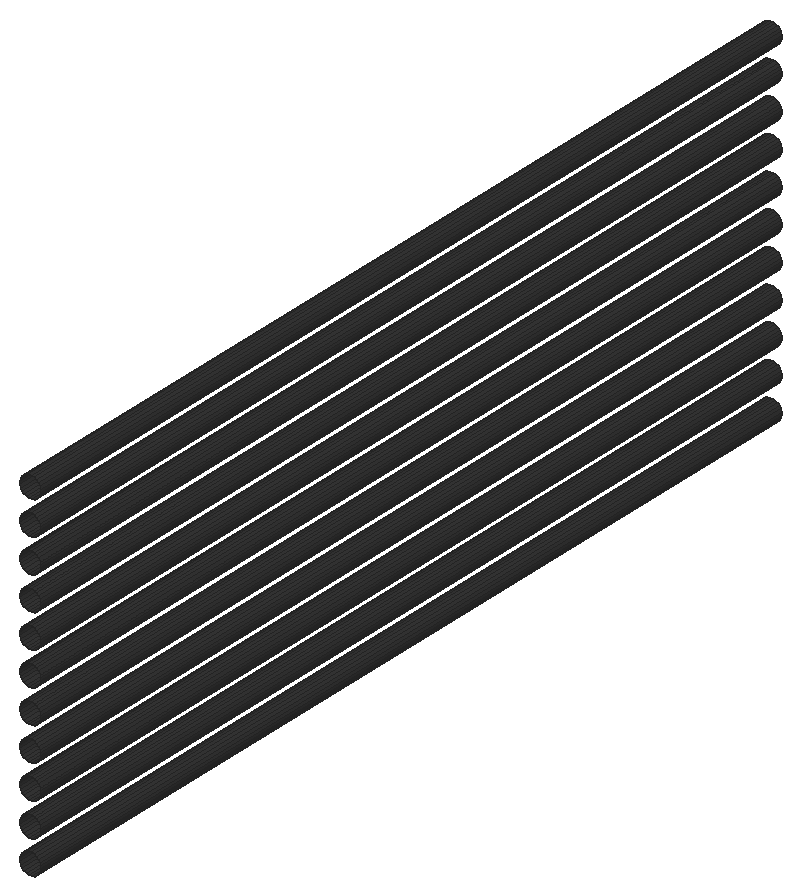
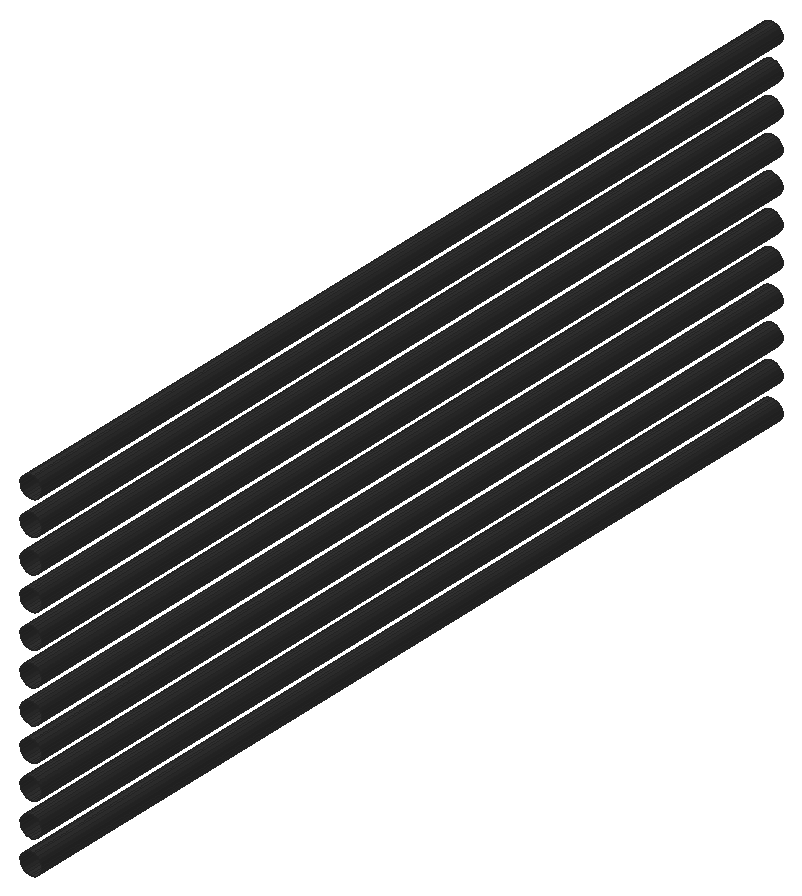
# SketchUp Ruby script. Lengths in inches.
U = 1.inch
M = Sketchup.active_model
def pt(a) = Geom::Point3d.new(a.map { |v| v * U })
def face(e, loops, mat)
  f = e.add_face(loops[0].map { |a| pt(a) })
  loops[1..].each { |l| e.add_face(l.map { |a| pt(a) }).erase! }
  f.material = f.back_material = mat if mat
  f
end
# faces: each face lists its corners as indices into pts; further lists are holes
def faces(e, pts, list, mat = nil) = list.each { |f| face(e, (f[0].is_a?(Array) ? f : [f]).map { |l| l.map { |i| pts[i] } }, mat) }
# xy, xz, yz: faces in a plane at the given z, y or x. An outline is a flat list of corners, or four numbers for a rectangle; further outlines are holes
def ring(l) = l.size == 4 ? [[l[0], l[1]], [l[2], l[1]], [l[2], l[3]], [l[0], l[3]]] : l.each_slice(2).to_a
def flat(e, list, mat, &to3) = list.each { |f| face(e, (f[0].is_a?(Array) ? f : [f]).map { |l| ring(l).map { |u, v| to3.(u, v) } }, mat) }
def xy(e, z, list, mat = nil) = flat(e, list, mat) { |x, y| [x, y, z] }
def xz(e, y, list, mat = nil) = flat(e, list, mat) { |x, z| [x, y, z] }
def yz(e, x, list, mat = nil) = flat(e, list, mat) { |y, z| [x, y, z] }
def lines(e, pts, list) = list.each { |a, b| e.add_line(pt(pts[a]), pt(pts[b])) }
# prism: a flat outline (further loops are holes) pulled along v
def prism(e, loops, v, mat = nil)
  f = face(e, loops, mat); d = Geom::Vector3d.new(v.map { |x| x * U })
  f.pushpull(f.normal.samedirection?(d) ? d.length : -d.length)
end
def box(e, o, s, mat = nil) = prism(e, [[o, [o[0] + s[0], o[1], o[2]], [o[0] + s[0], o[1] + s[1], o[2]], [o[0], o[1] + s[1], o[2]]]], [0, 0, s[2]], mat)
def at(x, y, z, deg = 0) = Geom::Transformation.translation(pt([x, y, z])) * Geom::Transformation.rotation(ORIGIN, Z_AXIS, deg.degrees)
def axes(o, x, y, z) = Geom::Transformation.new([*x, 0, *y, 0, *z, 0, *pt(o).to_a, 1])
def part(name) = M.definitions.add(name)
# library, detail: a bought-in or finely detailed component or shape, given as its bounding box
def library(name, o, s) = part(name).tap { |d| box(d.entities, o, s) }
def detail(e, o, s) = box(e.add_group.entities, o, s)
def put(e, d, t, mat = nil) = e.add_instance(d, t).tap { |i| i.material = mat if mat }
def group(e, t, mat = nil) = e.add_group.tap { |g| g.transformation = t; g.material = mat if mat }.entities
root = M.entities
M.materials.add("[0135_DarkGray]1").color = [53, 53, 53]
xy(root,397.39,[[1035.97,1165.35,1036.3125,1278.6875]],"[0135_DarkGray]1")
xy(root,405.66,[[1035.97,1165.35,1036.3125,1278.6875]],"[0135_DarkGray]1")
xy(root,408.26,[[1035.96,1165.35,1036.3,1278.6875]],"[0135_DarkGray]1")
xy(root,409.79,[[1035.97,1165.35,1036.3125,1278.6875]],"[0135_DarkGray]1")
xy(root,416.53,[[1035.96,1165.35,1036.3,1278.6875]],"[0135_DarkGray]1")
xy(root,418.06,[[1035.97,1165.35,1036.3125,1278.6875]],"[0135_DarkGray]1")
xy(root,420.66,[[1035.96,1165.35,1036.3,1278.6875]],"[0135_DarkGray]1")
xy(root,422.19,[[1035.97,1165.35,1036.3125,1278.6875]],"[0135_DarkGray]1")
xy(root,428.93,[[1035.96,1165.35,1036.3,1278.6875]],"[0135_DarkGray]1")
xy(root,430.46,[[1035.97,1165.35,1036.3125,1278.6875]],"[0135_DarkGray]1")
xy(root,434.59,[[1035.97,1165.35,1036.3125,1278.6875]],"[0135_DarkGray]1")
xy(root,441.33,[[1035.96,1165.35,1036.3,1278.6875]],"[0135_DarkGray]1")
yz(root,1034.83,[[1165.35,398.51,1278.6875,398.86],[1165.35,402.65,1278.6875,402.99],[1165.35,406.78,1278.6875,407.125],[1165.35,410.91,1278.6875,411.26],[1165.35,415.05,1278.6875,415.39],
  [1165.35,419.18,1278.6875,419.52],[1165.35,423.3125,1278.6875,423.66],[1165.35,427.45,1278.6875,427.79],[1165.35,431.58,1278.6875,431.92],[1165.35,435.71,1278.6875,436.06],
  [1165.35,439.85,1278.6875,440.19]],"[0135_DarkGray]1")
p = [[1035.97,1165.35,397.39],[1035.64,1165.35,397.48],[1035.64,1278.6875,397.48],[1035.97,1278.6875,397.39],[1036.64,1165.35,397.48],[1036.3125,1165.35,397.39],
  [1036.3125,1278.6875,397.39],[1036.64,1278.6875,397.48],[1035.34,1165.35,397.65],[1035.34,1278.6875,397.65],[1036.94,1165.35,397.66],[1036.94,1278.6875,397.66],
  [1035.1,1165.35,397.89],[1035.1,1278.6875,397.89],[1037.18,1165.35,397.9],[1037.18,1278.6875,397.9],[1034.93,1165.35,398.18],[1034.93,1278.6875,398.18],
  [1037.35,1165.35,398.2],[1037.35,1278.6875,398.2],[1034.83,1165.35,398.51],[1034.83,1278.6875,398.51],[1037.4375,1165.35,398.53],[1037.4375,1278.6875,398.53],
  [1037.44,1165.35,398.87],[1037.44,1278.6875,398.87],[1034.83,1165.35,398.86],[1034.92,1165.35,399.1875],[1034.92,1278.6875,399.1875],[1034.83,1278.6875,398.86],
  [1037.34,1165.35,399.2],[1037.34,1278.6875,399.2],[1035.09,1165.35,399.49],[1035.09,1278.6875,399.49],[1037.17,1165.35,399.5],[1037.17,1278.6875,399.5],
  [1035.33,1165.35,399.73],[1035.33,1278.6875,399.73],[1036.93,1165.35,399.74],[1036.93,1278.6875,399.74],[1035.625,1165.35,399.9],[1035.625,1278.6875,399.9],
  [1036.63,1165.35,399.91],[1036.63,1278.6875,399.91],[1035.96,1165.35,399.99],[1035.96,1278.6875,399.99],[1036.3,1165.35,400],[1036.3,1278.6875,400],
  [1035.97,1165.35,401.52],[1035.64,1165.35,401.61],[1035.64,1278.6875,401.61],[1035.97,1278.6875,401.52],[1036.3125,1165.35,401.53],[1036.3125,1278.6875,401.53],
  [1036.64,1165.35,401.62],[1036.64,1278.6875,401.62],[1035.34,1165.35,401.78],[1035.34,1278.6875,401.78],[1036.94,1165.35,401.79],[1036.94,1278.6875,401.79],
  [1035.1,1165.35,402.02],[1035.1,1278.6875,402.02],[1037.18,1165.35,402.03],[1037.18,1278.6875,402.03],[1034.93,1165.35,402.32],[1034.93,1278.6875,402.32],
  [1037.35,1165.35,402.33],[1037.35,1278.6875,402.33],[1034.83,1165.35,402.65],[1034.83,1278.6875,402.65],[1037.4375,1165.35,402.66],[1037.4375,1278.6875,402.66],
  [1037.44,1165.35,403],[1037.44,1278.6875,403],[1034.83,1165.35,402.99],[1034.92,1165.35,403.32],[1034.92,1278.6875,403.32],[1034.83,1278.6875,402.99],
  [1037.34,1165.35,403.34],[1037.34,1278.6875,403.34],[1035.09,1165.35,403.62],[1035.09,1278.6875,403.62],[1037.17,1165.35,403.63],[1037.17,1278.6875,403.63],
  [1035.33,1165.35,403.86],[1035.33,1278.6875,403.86],[1036.93,1165.35,403.87],[1036.93,1278.6875,403.87],[1035.625,1165.35,404.04],[1035.625,1278.6875,404.04],
  [1036.63,1165.35,404.04],[1036.63,1278.6875,404.04],[1035.96,1165.35,404.125],[1035.96,1278.6875,404.125],[1036.3,1165.35,404.13],[1036.3,1278.6875,404.13],
  [1035.64,1165.35,405.74],[1035.34,1165.35,405.91],[1035.34,1278.6875,405.91],[1035.64,1278.6875,405.74],[1035.97,1165.35,405.66],[1035.97,1278.6875,405.66],
  [1036.64,1165.35,405.75],[1036.3125,1165.35,405.66],[1036.3125,1278.6875,405.66],[1036.64,1278.6875,405.75],[1036.94,1165.35,405.92],[1036.94,1278.6875,405.92],
  [1035.1,1165.35,406.15],[1035.1,1278.6875,406.15],[1037.18,1165.35,406.17],[1037.18,1278.6875,406.17],[1034.93,1165.35,406.45],[1034.93,1278.6875,406.45],
  [1037.35,1165.35,406.46],[1037.35,1278.6875,406.46],[1034.83,1165.35,406.78],[1034.83,1278.6875,406.78],[1037.4375,1165.35,406.8],[1037.4375,1278.6875,406.8],
  [1037.44,1165.35,407.14],[1037.44,1278.6875,407.14],[1034.83,1165.35,407.125],[1034.92,1165.35,407.45],[1034.92,1278.6875,407.45],[1034.83,1278.6875,407.125],
  [1037.34,1165.35,407.47],[1037.34,1278.6875,407.47],[1035.09,1165.35,407.75],[1035.09,1278.6875,407.75],[1037.17,1165.35,407.76],[1037.17,1278.6875,407.76],
  [1035.33,1165.35,408],[1035.33,1278.6875,408],[1036.93,1165.35,408.01],[1036.93,1278.6875,408.01],[1035.625,1165.35,408.17],[1035.625,1278.6875,408.17],
  [1036.63,1165.35,408.17],[1036.63,1278.6875,408.17],[1035.96,1165.35,408.26],[1035.96,1278.6875,408.26],[1036.3,1165.35,408.26],[1036.3,1278.6875,408.26],
  [1035.97,1165.35,409.79],[1035.64,1165.35,409.88],[1035.64,1278.6875,409.88],[1035.97,1278.6875,409.79],[1036.64,1165.35,409.88],[1036.3125,1165.35,409.79],
  [1036.3125,1278.6875,409.79],[1036.64,1278.6875,409.88],[1035.34,1165.35,410.05],[1035.34,1278.6875,410.05],[1036.94,1165.35,410.06],[1036.94,1278.6875,410.06],
  [1035.1,1165.35,410.29],[1035.1,1278.6875,410.29],[1037.18,1165.35,410.3],[1037.18,1278.6875,410.3],[1034.93,1165.35,410.58],[1034.93,1278.6875,410.58],
  [1037.35,1165.35,410.6],[1037.35,1278.6875,410.6],[1034.83,1165.35,410.91],[1034.83,1278.6875,410.91],[1037.4375,1165.35,410.93],[1037.4375,1278.6875,410.93],
  [1037.44,1165.35,411.27],[1037.44,1278.6875,411.27],[1034.83,1165.35,411.26],[1034.92,1165.35,411.59],[1034.92,1278.6875,411.59],[1034.83,1278.6875,411.26],
  [1037.34,1165.35,411.6],[1037.34,1278.6875,411.6],[1035.09,1165.35,411.89],[1035.09,1278.6875,411.89],[1037.17,1165.35,411.9],[1037.17,1278.6875,411.9],
  [1035.33,1165.35,412.13],[1035.33,1278.6875,412.13],[1036.93,1165.35,412.14],[1036.93,1278.6875,412.14],[1035.625,1165.35,412.3],[1035.625,1278.6875,412.3],
  [1036.63,1165.35,412.31],[1036.63,1278.6875,412.31],[1035.96,1165.35,412.39],[1035.96,1278.6875,412.39],[1036.3,1165.35,412.4],[1036.3,1278.6875,412.4],
  [1035.97,1165.35,413.92],[1035.64,1165.35,414.01],[1035.64,1278.6875,414.01],[1035.97,1278.6875,413.92],[1036.3125,1165.35,413.93],[1036.3125,1278.6875,413.93],
  [1036.64,1165.35,414.02],[1036.64,1278.6875,414.02],[1035.34,1165.35,414.18],[1035.34,1278.6875,414.18],[1036.94,1165.35,414.1875],[1036.94,1278.6875,414.1875],
  [1035.1,1165.35,414.42],[1035.1,1278.6875,414.42],[1037.18,1165.35,414.43],[1037.18,1278.6875,414.43],[1034.93,1165.35,414.72],[1034.93,1278.6875,414.72],
  [1037.35,1165.35,414.73],[1037.35,1278.6875,414.73],[1034.83,1165.35,415.05],[1034.83,1278.6875,415.05],[1037.4375,1165.35,415.0625],[1037.4375,1278.6875,415.0625],
  [1037.44,1165.35,415.4],[1037.44,1278.6875,415.4],[1034.83,1165.35,415.39],[1034.92,1165.35,415.72],[1034.92,1278.6875,415.72],[1034.83,1278.6875,415.39],
  [1037.34,1165.35,415.74],[1037.34,1278.6875,415.74],[1035.09,1165.35,416.02],[1035.09,1278.6875,416.02],[1037.17,1165.35,416.03],[1037.17,1278.6875,416.03],
  [1035.33,1165.35,416.26],[1035.33,1278.6875,416.26],[1036.93,1165.35,416.27],[1036.93,1278.6875,416.27],[1035.625,1165.35,416.4375],[1035.625,1278.6875,416.4375],
  [1036.63,1165.35,416.44],[1036.63,1278.6875,416.44],[1035.96,1165.35,416.53],[1035.96,1278.6875,416.53],[1036.3,1165.35,416.53],[1036.3,1278.6875,416.53],
  [1035.64,1165.35,418.14],[1035.34,1165.35,418.3125],[1035.34,1278.6875,418.3125],[1035.64,1278.6875,418.14],[1035.97,1165.35,418.06],[1035.97,1278.6875,418.06],
  [1036.64,1165.35,418.15],[1036.3125,1165.35,418.06],[1036.3125,1278.6875,418.06],[1036.64,1278.6875,418.15],[1036.94,1165.35,418.32],[1036.94,1278.6875,418.32],
  [1035.1,1165.35,418.55],[1035.1,1278.6875,418.55],[1037.18,1165.35,418.57],[1037.18,1278.6875,418.57],[1034.93,1165.35,418.85],[1034.93,1278.6875,418.85],
  [1037.35,1165.35,418.86],[1037.35,1278.6875,418.86],[1034.83,1165.35,419.18],[1034.83,1278.6875,419.18],[1037.4375,1165.35,419.2],[1037.4375,1278.6875,419.2],
  [1037.44,1165.35,419.54],[1037.44,1278.6875,419.54],[1034.83,1165.35,419.52],[1034.92,1165.35,419.85],[1034.92,1278.6875,419.85],[1034.83,1278.6875,419.52],
  [1037.34,1165.35,419.87],[1037.34,1278.6875,419.87],[1035.09,1165.35,420.15],[1035.09,1278.6875,420.15],[1037.17,1165.35,420.16],[1037.17,1278.6875,420.16],
  [1035.33,1165.35,420.4],[1035.33,1278.6875,420.4],[1036.93,1165.35,420.41],[1036.93,1278.6875,420.41],[1035.625,1165.35,420.57],[1035.625,1278.6875,420.57],
  [1036.63,1165.35,420.57],[1036.63,1278.6875,420.57],[1035.96,1165.35,420.66],[1035.96,1278.6875,420.66],[1036.3,1165.35,420.66],[1036.3,1278.6875,420.66],
  [1035.97,1165.35,422.19],[1035.64,1165.35,422.28],[1035.64,1278.6875,422.28],[1035.97,1278.6875,422.19],[1036.64,1165.35,422.28],[1036.3125,1165.35,422.19],
  [1036.3125,1278.6875,422.19],[1036.64,1278.6875,422.28],[1035.34,1165.35,422.45],[1035.34,1278.6875,422.45],[1036.94,1165.35,422.46],[1036.94,1278.6875,422.46],
  [1035.1,1165.35,422.6875],[1035.1,1278.6875,422.6875],[1037.18,1165.35,422.7],[1037.18,1278.6875,422.7],[1034.93,1165.35,422.98],[1034.93,1278.6875,422.98],
  [1037.35,1165.35,423],[1037.35,1278.6875,423],[1034.83,1165.35,423.3125],[1034.83,1278.6875,423.3125],[1037.4375,1165.35,423.33],[1037.4375,1278.6875,423.33],
  [1037.44,1165.35,423.67],[1037.44,1278.6875,423.67],[1034.83,1165.35,423.66],[1034.92,1165.35,423.99],[1034.92,1278.6875,423.99],[1034.83,1278.6875,423.66],
  [1037.34,1165.35,424],[1037.34,1278.6875,424],[1035.09,1165.35,424.29],[1035.09,1278.6875,424.29],[1037.17,1165.35,424.3],[1037.17,1278.6875,424.3],
  [1035.33,1165.35,424.53],[1035.33,1278.6875,424.53],[1036.93,1165.35,424.54],[1036.93,1278.6875,424.54],[1035.625,1165.35,424.7],[1035.625,1278.6875,424.7],
  [1036.63,1165.35,424.71],[1036.63,1278.6875,424.71],[1035.96,1165.35,424.79],[1035.96,1278.6875,424.79],[1036.3,1165.35,424.8],[1036.3,1278.6875,424.8],
  [1035.97,1165.35,426.32],[1035.64,1165.35,426.41],[1035.64,1278.6875,426.41],[1035.97,1278.6875,426.32],[1036.3125,1165.35,426.33],[1036.3125,1278.6875,426.33],
  [1036.64,1165.35,426.42],[1036.64,1278.6875,426.42],[1035.34,1165.35,426.58],[1035.34,1278.6875,426.58],[1036.94,1165.35,426.59],[1036.94,1278.6875,426.59],
  [1035.1,1165.35,426.82],[1035.1,1278.6875,426.82],[1037.18,1165.35,426.83],[1037.18,1278.6875,426.83],[1034.93,1165.35,427.12],[1034.93,1278.6875,427.12],
  [1037.35,1165.35,427.13],[1037.35,1278.6875,427.13],[1034.83,1165.35,427.45],[1034.83,1278.6875,427.45],[1037.4375,1165.35,427.46],[1037.4375,1278.6875,427.46],
  [1037.44,1165.35,427.8],[1037.44,1278.6875,427.8],[1034.83,1165.35,427.79],[1034.92,1165.35,428.12],[1034.92,1278.6875,428.12],[1034.83,1278.6875,427.79],
  [1037.34,1165.35,428.14],[1037.34,1278.6875,428.14],[1035.09,1165.35,428.42],[1035.09,1278.6875,428.42],[1037.17,1165.35,428.43],[1037.17,1278.6875,428.43],
  [1035.33,1165.35,428.66],[1035.33,1278.6875,428.66],[1036.93,1165.35,428.67],[1036.93,1278.6875,428.67],[1035.625,1165.35,428.84],[1035.625,1278.6875,428.84],
  [1036.63,1165.35,428.84],[1036.63,1278.6875,428.84],[1035.96,1165.35,428.93],[1035.96,1278.6875,428.93],[1036.3,1165.35,428.93],[1036.3,1278.6875,428.93],
  [1035.64,1165.35,430.54],[1035.34,1165.35,430.71],[1035.34,1278.6875,430.71],[1035.64,1278.6875,430.54],[1035.97,1165.35,430.46],[1035.97,1278.6875,430.46],
  [1036.64,1165.35,430.55],[1036.3125,1165.35,430.46],[1036.3125,1278.6875,430.46],[1036.64,1278.6875,430.55],[1036.94,1165.35,430.72],[1036.94,1278.6875,430.72],
  [1035.1,1165.35,430.95],[1035.1,1278.6875,430.95],[1037.18,1165.35,430.97],[1037.18,1278.6875,430.97],[1034.93,1165.35,431.25],[1034.93,1278.6875,431.25],
  [1037.35,1165.35,431.26],[1037.35,1278.6875,431.26],[1034.83,1165.35,431.58],[1034.83,1278.6875,431.58],[1037.4375,1165.35,431.6],[1037.4375,1278.6875,431.6],
  [1037.44,1165.35,431.9375],[1037.44,1278.6875,431.9375],[1034.83,1165.35,431.92],[1034.92,1165.35,432.25],[1034.92,1278.6875,432.25],[1034.83,1278.6875,431.92],
  [1037.34,1165.35,432.27],[1037.34,1278.6875,432.27],[1035.09,1165.35,432.55],[1035.09,1278.6875,432.55],[1037.17,1165.35,432.5625],[1037.17,1278.6875,432.5625],
  [1035.33,1165.35,432.8],[1035.33,1278.6875,432.8],[1036.93,1165.35,432.81],[1036.93,1278.6875,432.81],[1035.625,1165.35,432.97],[1035.625,1278.6875,432.97],
  [1036.63,1165.35,432.97],[1036.63,1278.6875,432.97],[1035.96,1165.35,433.06],[1035.96,1278.6875,433.06],[1036.3,1165.35,433.0625],[1036.3,1278.6875,433.0625],
  [1035.97,1165.35,434.59],[1035.64,1165.35,434.68],[1035.64,1278.6875,434.68],[1035.97,1278.6875,434.59],[1036.64,1165.35,434.68],[1036.3125,1165.35,434.59],
  [1036.3125,1278.6875,434.59],[1036.64,1278.6875,434.68],[1035.34,1165.35,434.85],[1035.34,1278.6875,434.85],[1036.94,1165.35,434.86],[1036.94,1278.6875,434.86],
  [1035.1,1165.35,435.09],[1035.1,1278.6875,435.09],[1037.18,1165.35,435.1],[1037.18,1278.6875,435.1],[1034.93,1165.35,435.38],[1034.93,1278.6875,435.38],
  [1037.35,1165.35,435.4],[1037.35,1278.6875,435.4],[1034.83,1165.35,435.71],[1034.83,1278.6875,435.71],[1037.4375,1165.35,435.73],[1037.4375,1278.6875,435.73],
  [1037.44,1165.35,436.07],[1037.44,1278.6875,436.07],[1034.83,1165.35,436.06],[1034.92,1165.35,436.39],[1034.92,1278.6875,436.39],[1034.83,1278.6875,436.06],
  [1037.34,1165.35,436.4],[1037.34,1278.6875,436.4],[1035.09,1165.35,436.6875],[1035.09,1278.6875,436.6875],[1037.17,1165.35,436.7],[1037.17,1278.6875,436.7],
  [1035.33,1165.35,436.93],[1035.33,1278.6875,436.93],[1036.93,1165.35,436.9375],[1036.93,1278.6875,436.9375],[1035.625,1165.35,437.1],[1035.625,1278.6875,437.1],
  [1036.63,1165.35,437.11],[1036.63,1278.6875,437.11],[1035.96,1165.35,437.19],[1035.96,1278.6875,437.19],[1036.3,1165.35,437.2],[1036.3,1278.6875,437.2],
  [1035.97,1165.35,438.72],[1035.64,1165.35,438.8125],[1035.64,1278.6875,438.8125],[1035.97,1278.6875,438.72],[1036.3125,1165.35,438.73],[1036.3125,1278.6875,438.73],
  [1036.64,1165.35,438.82],[1036.64,1278.6875,438.82],[1035.34,1165.35,438.98],[1035.34,1278.6875,438.98],[1036.94,1165.35,438.99],[1036.94,1278.6875,438.99],
  [1035.1,1165.35,439.22],[1035.1,1278.6875,439.22],[1037.18,1165.35,439.23],[1037.18,1278.6875,439.23],[1034.93,1165.35,439.52],[1034.93,1278.6875,439.52],
  [1037.35,1165.35,439.53],[1037.35,1278.6875,439.53],[1034.83,1165.35,439.85],[1034.83,1278.6875,439.85],[1037.4375,1165.35,439.86],[1037.4375,1278.6875,439.86],
  [1037.44,1165.35,440.2],[1037.44,1278.6875,440.2],[1034.83,1165.35,440.19],[1034.92,1165.35,440.52],[1034.92,1278.6875,440.52],[1034.83,1278.6875,440.19],
  [1037.34,1165.35,440.54],[1037.34,1278.6875,440.54],[1035.09,1165.35,440.82],[1035.09,1278.6875,440.82],[1037.17,1165.35,440.83],[1037.17,1278.6875,440.83],
  [1035.33,1165.35,441.0625],[1035.33,1278.6875,441.0625],[1036.93,1165.35,441.07],[1036.93,1278.6875,441.07],[1035.625,1165.35,441.24],[1035.625,1278.6875,441.24],
  [1036.63,1165.35,441.24],[1036.63,1278.6875,441.24],[1035.96,1165.35,441.33],[1035.96,1278.6875,441.33],[1036.3,1165.35,441.33],[1036.3,1278.6875,441.33]]
faces(root,p,[[0,1,2,3],[4,5,6,7],[1,8,9,2],[10,4,7,11],[8,12,13,9],[14,10,11,15],[12,16,17,13],[18,14,15,19],
  [16,20,21,17],[22,18,19,23],[24,22,23,25],[26,27,28,29],[30,24,25,31],[27,32,33,28],[34,30,31,35],[32,36,37,33],
  [38,34,35,39],[36,40,41,37],[42,38,39,43],[40,44,45,41],[46,42,43,47],[44,46,47,45],[48,49,50,51],[52,48,51,53],
  [54,52,53,55],[49,56,57,50],[58,54,55,59],[56,60,61,57],[62,58,59,63],[60,64,65,61],[66,62,63,67],[64,68,69,65],
  [70,66,67,71],[72,70,71,73],[74,75,76,77],[78,72,73,79],[75,80,81,76],[82,78,79,83],[80,84,85,81],[86,82,83,87],
  [84,88,89,85],[90,86,87,91],[88,92,93,89],[94,90,91,95],[92,94,95,93],[96,97,98,99],[100,96,99,101],[102,103,104,105],
  [106,102,105,107],[97,108,109,98],[110,106,107,111],[108,112,113,109],[114,110,111,115],[112,116,117,113],[118,114,115,119],[120,118,119,121],
  [122,123,124,125],[126,120,121,127],[123,128,129,124],[130,126,127,131],[128,132,133,129],[134,130,131,135],[132,136,137,133],[138,134,135,139],
  [136,140,141,137],[142,138,139,143],[144,145,146,147],[148,149,150,151],[145,152,153,146],[154,148,151,155],[152,156,157,153],[158,154,155,159],
  [156,160,161,157],[162,158,159,163],[160,164,165,161],[166,162,163,167],[168,166,167,169],[170,171,172,173],[174,168,169,175],[171,176,177,172],
  [178,174,175,179],[176,180,181,177],[182,178,179,183],[180,184,185,181],[186,182,183,187],[184,188,189,185],[190,186,187,191],[188,190,191,189],
  [192,193,194,195],[196,192,195,197],[198,196,197,199],[193,200,201,194],[202,198,199,203],[200,204,205,201],[206,202,203,207],[204,208,209,205],
  [210,206,207,211],[208,212,213,209],[214,210,211,215],[216,214,215,217],[218,219,220,221],[222,216,217,223],[219,224,225,220],[226,222,223,227],
  [224,228,229,225],[230,226,227,231],[228,232,233,229],[234,230,231,235],[232,236,237,233],[238,234,235,239],[240,241,242,243],[244,240,243,245],
  [246,247,248,249],[250,246,249,251],[241,252,253,242],[254,250,251,255],[252,256,257,253],[258,254,255,259],[256,260,261,257],[262,258,259,263],
  [264,262,263,265],[266,267,268,269],[270,264,265,271],[267,272,273,268],[274,270,271,275],[272,276,277,273],[278,274,275,279],[276,280,281,277],
  [282,278,279,283],[280,284,285,281],[286,282,283,287],[288,289,290,291],[292,293,294,295],[289,296,297,290],[298,292,295,299],[296,300,301,297],
  [302,298,299,303],[300,304,305,301],[306,302,303,307],[304,308,309,305],[310,306,307,311],[312,310,311,313],[314,315,316,317],[318,312,313,319],
  [315,320,321,316],[322,318,319,323],[320,324,325,321],[326,322,323,327],[324,328,329,325],[330,326,327,331],[328,332,333,329],[334,330,331,335],
  [332,334,335,333],[336,337,338,339],[340,336,339,341],[342,340,341,343],[337,344,345,338],[346,342,343,347],[344,348,349,345],[350,346,347,351],
  [348,352,353,349],[354,350,351,355],[352,356,357,353],[358,354,355,359],[360,358,359,361],[362,363,364,365],[366,360,361,367],[363,368,369,364],
  [370,366,367,371],[368,372,373,369],[374,370,371,375],[372,376,377,373],[378,374,375,379],[376,380,381,377],[382,378,379,383],[384,385,386,387],
  [388,384,387,389],[390,391,392,393],[394,390,393,395],[385,396,397,386],[398,394,395,399],[396,400,401,397],[402,398,399,403],[400,404,405,401],
  [406,402,403,407],[408,406,407,409],[410,411,412,413],[414,408,409,415],[411,416,417,412],[418,414,415,419],[416,420,421,417],[422,418,419,423],
  [420,424,425,421],[426,422,423,427],[424,428,429,425],[430,426,427,431],[428,430,431,429],[432,433,434,435],[436,437,438,439],[433,440,441,434],
  [442,436,439,443],[440,444,445,441],[446,442,443,447],[444,448,449,445],[450,446,447,451],[448,452,453,449],[454,450,451,455],[456,454,455,457],
  [458,459,460,461],[462,456,457,463],[459,464,465,460],[466,462,463,467],[464,468,469,465],[470,466,467,471],[468,472,473,469],[474,470,471,475],
  [472,476,477,473],[478,474,475,479],[476,478,479,477],[480,481,482,483],[484,480,483,485],[486,484,485,487],[481,488,489,482],[490,486,487,491],
  [488,492,493,489],[494,490,491,495],[492,496,497,493],[498,494,495,499],[496,500,501,497],[502,498,499,503],[504,502,503,505],[506,507,508,509],
  [510,504,505,511],[507,512,513,508],[514,510,511,515],[512,516,517,513],[518,514,515,519],[516,520,521,517],[522,518,519,523],[520,524,525,521],
  [526,522,523,527]],"[0135_DarkGray]1")
